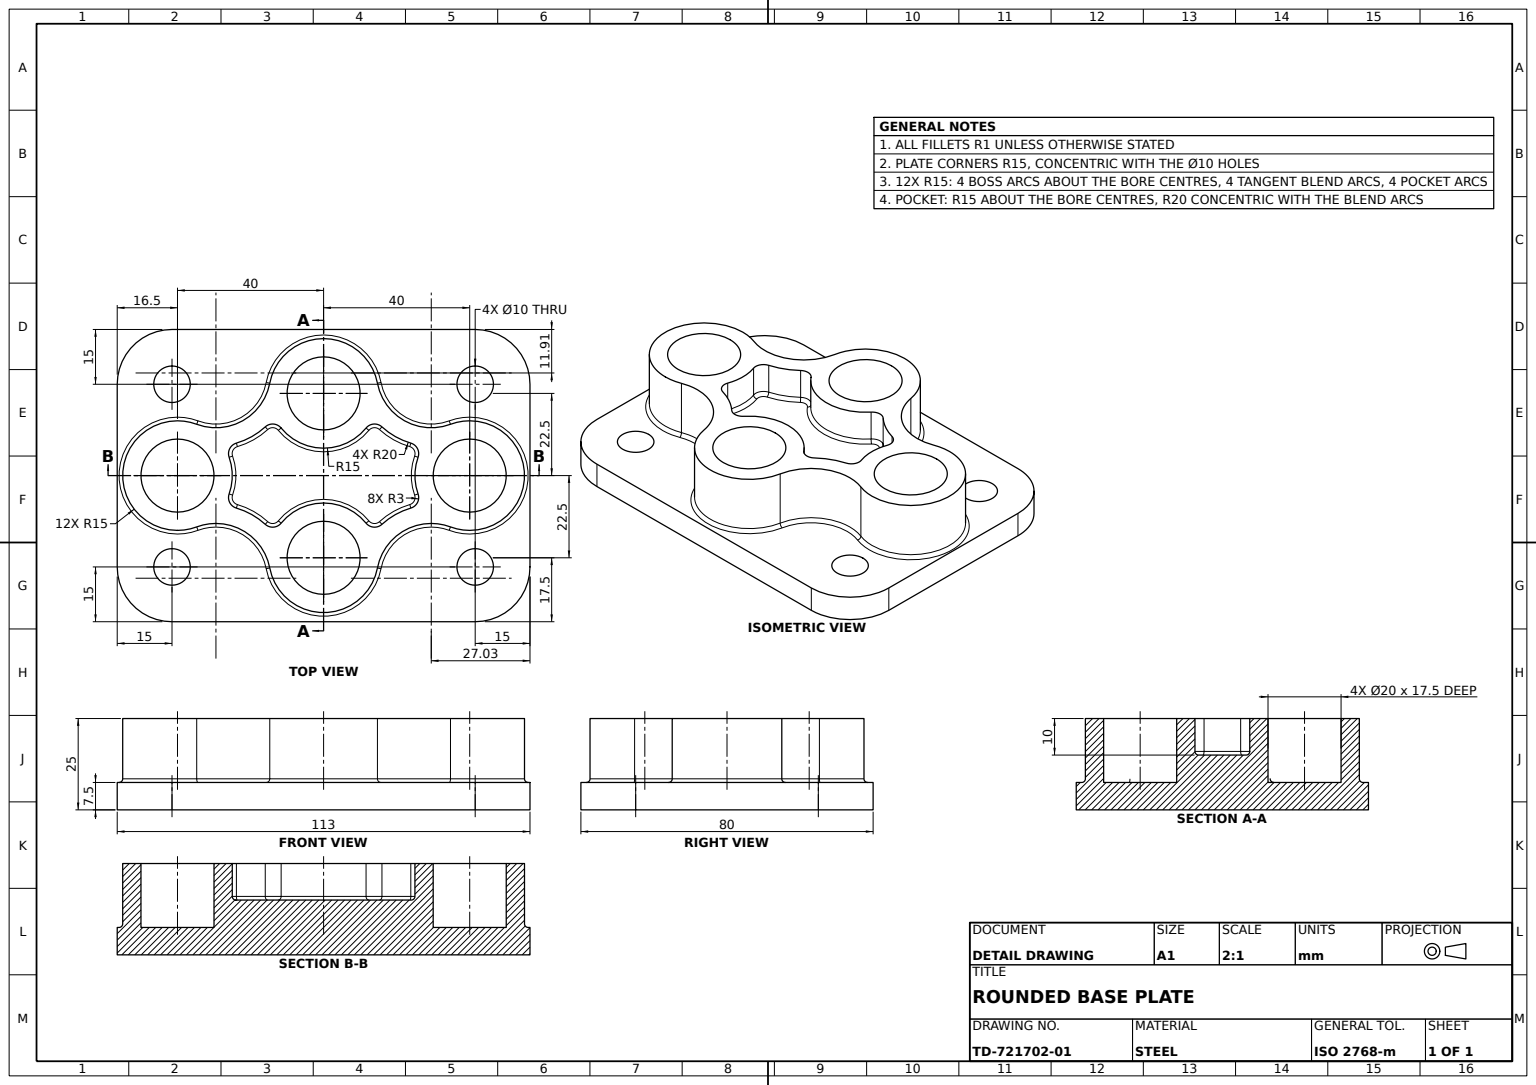
solid
v1 (-29.474069,1,13.092789)
v2 (-14.737034,1,25.296394)
e1 v1 v2 CIRCLE(AX(P(-29.474069,1,28.092789),D(0,-1,0),D(0,0,-1)),15)
v3 (-29.474069,0,14.092789)
e2 v1 v3 CIRCLE(AX(P(-29.474069,1,14.092789),D(-1,0,0),D(0,0,1)),1)
v4 (-15.719503,0,25.482821)
e3 v4 v3 CIRCLE(AX(P(-29.474069,0,28.092789),D(0,1,0),D(0,0,-1)),14)
e4 v4 v2 CIRCLE(AX(P(-15.719503,1,25.482821),D(0.186426284,0,0.982468951),D(0.982468951,0,-0.186426284)),1)
face TORUS(AX(P(-29.474069,1,28.092789),D(0,-1,0),D(0,0,-1)),14,1) rev [-e1 e2 -e3 e4]
v5 (40,1,-15)
v6 (34.737034,1,-14.046394)
e5 v5 v6 CIRCLE(AX(P(40,1,0),D(0,1,0),D(0,0,-1)),15)
v7 (34.737034,17.5,-14.046394)
e6 v7 v6 LINE
v8 (40,17.5,-15)
e7 v8 v7 CIRCLE(AX(P(40,17.5,0),D(0,1,0),D(0,0,-1)),15)
e8 v8 v5 LINE
face CYL(AX(P(40,17.5,0),D(0,-1,0),D(0,0,-1)),15) [e5 -e6 -e7 e8]
v9 (-34.737034,1,-14.046394)
v10 (-40,1,-15)
e9 v9 v10 CIRCLE(AX(P(-40,1,0),D(0,1,0),D(0,0,-1)),15)
v11 (-34.38617,0,-14.982821)
e10 v9 v11 CIRCLE(AX(P(-34.38617,1,-14.982821),D(0.936426284,0,0.350864382),D(0.350864382,0,-0.936426284)),1)
v12 (-40,0,-16)
e11 v12 v11 CIRCLE(AX(P(-40,0,0),D(0,-1,0),D(0,0,-1)),16)
e12 v12 v10 CIRCLE(AX(P(-40,1,-16),D(-1,0,0),D(0,0,1)),1)
face TORUS(AX(P(-40,1,0),D(0,-1,0),D(0,0,-1)),16,1) rev [-e9 e10 -e11 e12]
v13 (15.298823,7.5,-12.598841)
v14 (12.398933,7.5,-12.387312)
e13 v13 v14 CIRCLE(AX(P(13.9488,7.5,-11.123226),D(0,1,0),D(0,0,1)),2)
v15 (15.973835,8.5,-13.336648)
e14 v13 v15 CIRCLE(AX(P(15.298823,8.5,-12.598841),D(0.737807048,0,0.675011674),D(0.675011674,0,-0.737807048)),1)
v16 (13.9488,8.5,-14.123226)
e15 v16 v15 CIRCLE(AX(P(13.9488,8.5,-11.123226),D(0,-1,0),D(0,0,1)),3)
v17 (11.624,8.5,-13.019355)
e16 v17 v16 CIRCLE(AX(P(13.9488,8.5,-11.123226),D(0,-1,0),D(0,0,1)),3)
e17 v14 v17 CIRCLE(AX(P(12.398933,8.5,-12.387312),D(0.632042977,0,-0.774933336),D(-0.774933336,0,-0.632042977)),1)
face TORUS(AX(P(13.9488,8.5,-11.123226),D(0,1,0),D(0,0,1)),2,1) rev [-e13 e14 -e15 -e16 -e17]
v18 (14.737034,1,-25.296394)
v19 (15.719503,0,-25.482821)
e18 v18 v19 CIRCLE(AX(P(15.719503,1,-25.482821),D(0.186426284,0,0.982468951),D(0.982468951,0,-0.186426284)),1)
v20 (0,0,-38.5)
e19 v20 v19 CIRCLE(AX(P(0,0,-22.5),D(0,-1,0),D(0,0,-1)),16)
v21 (0,1,-37.5)
e20 v20 v21 CIRCLE(AX(P(0,1,-38.5),D(-1,0,0),D(0,0,1)),1)
e21 v18 v21 CIRCLE(AX(P(0,1,-22.5),D(0,1,0),D(0,0,-1)),15)
face TORUS(AX(P(0,1,-22.5),D(0,-1,0),D(0,0,-1)),16,1) rev [e18 -e19 e20 -e21]
v22 (-40,0,16)
e22 v22 v12 CIRCLE(AX(P(-40,0,0),D(0,-1,0),D(0,0,-1)),16)
v23 (-40,1,15)
e23 v22 v23 CIRCLE(AX(P(-40,1,16),D(1,0,0),D(0,0,-1)),1)
e24 v10 v23 CIRCLE(AX(P(-40,1,0),D(0,1,0),D(0,0,-1)),15)
face TORUS(AX(P(-40,1,0),D(0,-1,0),D(0,0,-1)),16,1) rev [-e22 e23 -e24 -e12]
v24 (-25.861645,17.5,-5.01068)
v25 (-25.861645,8.5,-5.01068)
e25 v24 v25 LINE
v26 (-25.861645,17.5,5.01068)
e26 v24 v26 CIRCLE(AX(P(-40,17.5,0),D(0,-1,0),D(0,0,1)),15)
v27 (-25.861645,8.5,5.01068)
e27 v26 v27 LINE
e28 v27 v25 CIRCLE(AX(P(-40,8.5,0),D(0,1,0),D(0,0,1)),15)
face CYL(AX(P(-40,17.5,0),D(0,-1,0),D(0,0,-1)),15) [-e25 e26 e27 e28]
v28 (40,17.5,15)
e29 v28 v8 CIRCLE(AX(P(40,17.5,0),D(0,1,0),D(0,0,-1)),15)
v29 (40,1,15)
e30 v28 v29 LINE
e31 v29 v5 CIRCLE(AX(P(40,1,0),D(0,1,0),D(0,0,-1)),15)
face CYL(AX(P(40,17.5,0),D(0,-1,0),D(0,0,-1)),15) [-e29 e30 e31 -e8]
v30 (56.5,0,25)
v31 (56.5,-7.5,25)
e32 v30 v31 LINE
v32 (41.5,0,40)
e33 v32 v30 CIRCLE(AX(P(41.5,0,25),D(0,1,0),D(0,0,-1)),15)
v33 (41.5,-7.5,40)
e34 v33 v32 LINE
e35 v31 v33 CIRCLE(AX(P(41.5,-7.5,25),D(0,-1,0),D(0,0,-1)),15)
face CYL(AX(P(41.5,-7.5,25),D(0,1,0),D(0,0,1)),15) [-e32 -e33 -e34 -e35]
v34 (23.593982,7.5,7.932814)
v35 (23.873986,8.5,8.892813)
e36 v34 v35 CIRCLE(AX(P(23.593982,8.5,7.932814),D(-0.9599988,0,0.280004116),D(0.280004116,0,0.9599988)),1)
v36 (25.861645,8.5,5.01068)
e37 v36 v35 CIRCLE(AX(P(23.033974,8.5,6.012816),D(0,-1,0),D(0,0,1)),3)
v37 (24.919088,7.5,5.344725)
e38 v37 v36 CIRCLE(AX(P(24.919088,8.5,5.344725),D(0.334045341,0,0.942557006),D(0.942557006,0,-0.334045341)),1)
e39 v34 v37 CIRCLE(AX(P(23.033974,7.5,6.012816),D(0,1,0),D(0,0,1)),2)
face TORUS(AX(P(23.033974,8.5,6.012816),D(0,1,0),D(0,0,1)),2,1) rev [e36 -e37 -e38 -e39]
v38 (15.719503,0,25.482821)
e40 v38 v4 CIRCLE(AX(P(0,0,22.5),D(0,-1,0),D(0,0,-1)),16)
v39 (14.737034,1,25.296394)
e41 v38 v39 CIRCLE(AX(P(15.719503,1,25.482821),D(0.186426284,0,-0.982468951),D(-0.982468951,0,-0.186426284)),1)
e42 v2 v39 CIRCLE(AX(P(0,1,22.5),D(0,1,0),D(0,0,-1)),15)
face TORUS(AX(P(0,1,22.5),D(0,-1,0),D(0,0,-1)),16,1) rev [-e40 e41 -e42 -e4]
v40 (0,17.5,-37.5)
v41 (-14.737034,17.5,-25.296394)
e43 v40 v41 CIRCLE(AX(P(0,17.5,-22.5),D(0,1,0),D(0,0,-1)),15)
e44 v40 v21 LINE
v42 (-14.737034,1,-25.296394)
e45 v21 v42 CIRCLE(AX(P(0,1,-22.5),D(0,1,0),D(0,0,-1)),15)
e46 v41 v42 LINE
face CYL(AX(P(0,17.5,-22.5),D(0,-1,0),D(0,0,-1)),15) [-e43 e44 e45 -e46]
v43 (-15.973835,8.5,-13.336648)
v44 (-13.9488,8.5,-14.123226)
e47 v43 v44 CIRCLE(AX(P(-13.9488,8.5,-11.123226),D(0,-1,0),D(0,0,1)),3)
v45 (-13.9488,17.5,-14.123226)
e48 v45 v44 LINE
v46 (-15.973835,17.5,-13.336648)
e49 v45 v46 CIRCLE(AX(P(-13.9488,17.5,-11.123226),D(0,1,0),D(0,0,1)),3)
e50 v46 v43 LINE
face CYL(AX(P(-13.9488,17.5,-11.123226),D(0,-1,0),D(0,0,-1)),3) rev [e47 -e48 e49 e50]
v47 (-23.873986,17.5,8.892813)
v48 (-23.873986,8.5,8.892813)
e51 v47 v48 LINE
v49 (-15.973835,17.5,13.336648)
e52 v47 v49 CIRCLE(AX(P(-29.474069,17.5,28.092789),D(0,-1,0),D(0,0,-1)),20)
v50 (-15.973835,8.5,13.336648)
e53 v49 v50 LINE
e54 v50 v48 CIRCLE(AX(P(-29.474069,8.5,28.092789),D(0,1,0),D(0,0,1)),20)
face CYL(AX(P(-29.474069,17.5,28.092789),D(0,-1,0),D(0,0,-1)),20) [-e51 e52 e53 e54]
v51 (-41.5,0,40)
e55 v51 v32 LINE
v52 (-41.5,-7.5,40)
e56 v51 v52 LINE
e57 v52 v33 LINE
face PLANE(AX(P(-56.5,-7.5,40),D(0,0,1),D(1,0,0))) [-e55 e56 e57 e34]
v53 (40,0,-16)
e58 v53 v5 CIRCLE(AX(P(40,1,-16),D(-1,0,0),D(0,0,1)),1)
v54 (40,0,16)
e59 v54 v29 CIRCLE(AX(P(40,1,16),D(1,0,0),D(0,0,-1)),1)
e60 v53 v54 CIRCLE(AX(P(40,0,0),D(0,-1,0),D(0,0,-1)),16)
face TORUS(AX(P(40,1,0),D(0,-1,0),D(0,0,-1)),16,1) rev [e58 -e31 -e59 -e60]
v55 (13.9488,17.5,-14.123226)
e61 v55 v16 LINE
v56 (11.624,17.5,-13.019355)
e62 v55 v56 CIRCLE(AX(P(13.9488,17.5,-11.123226),D(0,1,0),D(0,0,-1)),3)
e63 v56 v17 LINE
face CYL(AX(P(13.9488,17.5,-11.123226),D(0,-1,0),D(0,0,-1)),3) rev [e16 -e61 e62 e63]
v57 (-14.737034,17.5,25.296394)
e64 v57 v2 LINE
v58 (14.737034,17.5,25.296394)
e65 v58 v39 LINE
e66 v57 v58 CIRCLE(AX(P(0,17.5,22.5),D(0,1,0),D(0,0,1)),15)
face CYL(AX(P(0,17.5,22.5),D(0,-1,0),D(0,0,-1)),15) [e64 e42 -e65 -e66]
v59 (-29.474069,17.5,13.092789)
e67 v59 v57 CIRCLE(AX(P(-29.474069,17.5,28.092789),D(0,-1,0),D(0,0,-1)),15)
e68 v59 v1 LINE
face CYL(AX(P(-29.474069,17.5,28.092789),D(0,-1,0),D(0,0,-1)),15) rev [-e64 -e67 e68 e1]
v60 (34.737034,1,14.046394)
e69 v60 v29 CIRCLE(AX(P(40,1,0),D(0,1,0),D(0,0,-1)),15)
v61 (34.38617,0,14.982821)
e70 v61 v60 CIRCLE(AX(P(34.38617,1,14.982821),D(0.936426284,0,0.350864382),D(0.350864382,0,-0.936426284)),1)
e71 v54 v61 CIRCLE(AX(P(40,0,0),D(0,-1,0),D(0,0,-1)),16)
face TORUS(AX(P(40,1,0),D(0,-1,0),D(0,0,-1)),16,1) rev [-e69 -e70 -e71 e59]
v62 (0,0,-32.5)
v63 (0,0,-12.5)
e72 v62 v63 CIRCLE(AX(P(0,0,-22.5),D(0,1,0),D(0,0,-1)),10)
e73 v63 v62 CIRCLE(AX(P(0,0,-22.5),D(0,1,0),D(0,0,-1)),10)
face PLANE(AX(P(0,0,0),D(0,-1,0),D(0,0,-1))) rev [e72 e73]
v64 (-23.873986,8.5,-8.892813)
e74 v64 v43 CIRCLE(AX(P(-29.474069,8.5,-28.092789),D(0,1,0),D(0,0,1)),20)
v65 (-23.593982,7.5,-7.932814)
e75 v64 v65 CIRCLE(AX(P(-23.593982,8.5,-7.932814),D(-0.9599988,0,0.280004116),D(0.280004116,0,0.9599988)),1)
v66 (-15.298823,7.5,-12.598841)
e76 v66 v65 CIRCLE(AX(P(-29.474069,7.5,-28.092789),D(0,-1,0),D(0,0,1)),21)
e77 v43 v66 CIRCLE(AX(P(-15.298823,8.5,-12.598841),D(-0.737807048,0,0.675011674),D(0.675011674,0,0.737807048)),1)
face TORUS(AX(P(-29.474069,8.5,-28.092789),D(0,1,0),D(0,0,1)),21,1) rev [-e74 e75 -e76 -e77]
v67 (-41.5,0,-30)
v68 (-41.5,0,-20)
e78 v67 v68 CIRCLE(AX(P(-41.5,0,-25),D(0,1,0),D(0,0,1)),5)
v69 (-41.5,-7.5,-20)
e79 v69 v68 LINE
v70 (-41.5,-7.5,-30)
e80 v69 v70 CIRCLE(AX(P(-41.5,-7.5,-25),D(0,-1,0),D(0,0,-1)),5)
e81 v70 v67 LINE
face CYL(AX(P(-41.5,-17.5,-25),D(0,1,0),D(0,0,1)),5) rev [e78 -e79 e80 e81]
v71 (29.474069,1,13.092789)
e82 v39 v71 CIRCLE(AX(P(29.474069,1,28.092789),D(0,-1,0),D(0,0,-1)),15)
v72 (29.474069,17.5,13.092789)
e83 v72 v71 LINE
e84 v58 v72 CIRCLE(AX(P(29.474069,17.5,28.092789),D(0,-1,0),D(0,0,1)),15)
face CYL(AX(P(29.474069,17.5,28.092789),D(0,-1,0),D(0,0,-1)),15) rev [e82 -e83 -e84 e65]
v73 (40,0,10)
v74 (40,0,-10)
e85 v73 v74 CIRCLE(AX(P(40,0,0),D(0,1,0),D(0,0,-1)),10)
e86 v74 v73 CIRCLE(AX(P(40,0,0),D(0,1,0),D(0,0,-1)),10)
face PLANE(AX(P(0,0,0),D(0,-1,0),D(0,0,-1))) rev [e85 e86]
v75 (15.973835,17.5,13.336648)
v76 (15.973835,8.5,13.336648)
e87 v75 v76 LINE
v77 (23.873986,17.5,8.892813)
e88 v75 v77 CIRCLE(AX(P(29.474069,17.5,28.092789),D(0,-1,0),D(0,0,1)),20)
e89 v77 v35 LINE
e90 v35 v76 CIRCLE(AX(P(29.474069,8.5,28.092789),D(0,1,0),D(0,0,1)),20)
face CYL(AX(P(29.474069,17.5,28.092789),D(0,-1,0),D(0,0,-1)),20) [-e87 e88 e89 e90]
v78 (-24.919088,7.5,5.344725)
e91 v27 v78 CIRCLE(AX(P(-24.919088,8.5,5.344725),D(-0.334045341,0,0.942557006),D(0.942557006,0,0.334045341)),1)
v79 (-24.919088,7.5,-5.344725)
e92 v79 v78 CIRCLE(AX(P(-40,7.5,0),D(0,-1,0),D(0,0,1)),16)
e93 v25 v79 CIRCLE(AX(P(-24.919088,8.5,-5.344725),D(0.334045341,0,0.942557006),D(0.942557006,0,-0.334045341)),1)
face TORUS(AX(P(-40,8.5,0),D(0,1,0),D(0,0,1)),16,1) rev [e91 -e92 -e93 -e28]
v80 (15.298823,7.5,12.598841)
e94 v80 v76 CIRCLE(AX(P(15.298823,8.5,12.598841),D(-0.737807048,0,0.675011674),D(0.675011674,0,0.737807048)),1)
e95 v80 v34 CIRCLE(AX(P(29.474069,7.5,28.092789),D(0,-1,0),D(0,0,1)),21)
face TORUS(AX(P(29.474069,8.5,28.092789),D(0,1,0),D(0,0,1)),21,1) rev [e94 -e90 -e36 -e95]
v81 (-11.624,17.5,13.019355)
e96 v49 v81 CIRCLE(AX(P(-13.9488,17.5,11.123226),D(0,1,0),D(0,0,-1)),3)
v82 (-11.624,8.5,13.019355)
e97 v81 v82 LINE
v83 (-13.9488,8.5,14.123226)
e98 v82 v83 CIRCLE(AX(P(-13.9488,8.5,11.123226),D(0,-1,0),D(0,0,1)),3)
e99 v83 v50 CIRCLE(AX(P(-13.9488,8.5,11.123226),D(0,-1,0),D(0,0,1)),3)
face CYL(AX(P(-13.9488,17.5,11.123226),D(0,-1,0),D(0,0,-1)),3) rev [e96 e97 e98 e99 -e53]
v84 (41.5,-7.5,-20)
v85 (41.5,-7.5,-30)
e100 v84 v85 CIRCLE(AX(P(41.5,-7.5,-25),D(0,-1,0),D(0,0,-1)),5)
e101 v85 v84 CIRCLE(AX(P(41.5,-7.5,-25),D(0,-1,0),D(0,0,-1)),5)
v86 (41.5,-7.5,30)
v87 (41.5,-7.5,20)
e102 v86 v87 CIRCLE(AX(P(41.5,-7.5,25),D(0,-1,0),D(0,0,-1)),5)
e103 v87 v86 CIRCLE(AX(P(41.5,-7.5,25),D(0,-1,0),D(0,0,-1)),5)
v88 (-56.5,-7.5,-25)
v89 (-56.5,-7.5,25)
e104 v88 v89 LINE
v90 (-41.5,-7.5,-40)
e105 v88 v90 CIRCLE(AX(P(-41.5,-7.5,-25),D(0,-1,0),D(0,0,-1)),15)
v91 (41.5,-7.5,-40)
e106 v91 v90 LINE
v92 (56.5,-7.5,-25)
e107 v91 v92 CIRCLE(AX(P(41.5,-7.5,-25),D(0,-1,0),D(0,0,-1)),15)
e108 v31 v92 LINE
e109 v52 v89 CIRCLE(AX(P(-41.5,-7.5,25),D(0,-1,0),D(0,0,-1)),15)
v93 (-41.5,-7.5,30)
v94 (-41.5,-7.5,20)
e110 v93 v94 CIRCLE(AX(P(-41.5,-7.5,25),D(0,-1,0),D(0,0,-1)),5)
e111 v94 v93 CIRCLE(AX(P(-41.5,-7.5,25),D(0,-1,0),D(0,0,-1)),5)
e112 v70 v69 CIRCLE(AX(P(-41.5,-7.5,-25),D(0,-1,0),D(0,0,-1)),5)
face PLANE(AX(P(0,-7.5,0),D(0,-1,0),D(0,0,-1))) [-e100 -e101] [-e102 -e103] [-e104 e105 -e106 e107 -e108 e35 -e57 e109] [-e110 -e111] [-e112 -e80]
v95 (0,17.5,32.5)
v96 (0,17.5,12.5)
e113 v95 v96 CIRCLE(AX(P(0,17.5,22.5),D(0,1,0),D(0,0,1)),10)
v97 (0,0,12.5)
e114 v96 v97 LINE
v98 (0,0,32.5)
e115 v98 v97 CIRCLE(AX(P(0,0,22.5),D(0,1,0),D(0,0,1)),10)
e116 v95 v98 LINE
face CYL(AX(P(0,17.5,22.5),D(0,-1,0),D(0,0,-1)),10) rev [e113 e114 -e115 -e116]
v99 (-41.5,0,30)
e117 v93 v99 LINE
v100 (-41.5,0,20)
e118 v99 v100 CIRCLE(AX(P(-41.5,0,25),D(0,1,0),D(0,0,1)),5)
e119 v94 v100 LINE
face CYL(AX(P(-41.5,-17.5,25),D(0,1,0),D(0,0,1)),5) rev [e117 e118 -e119 e111]
v101 (24.919088,7.5,-5.344725)
v102 (25.861645,8.5,-5.01068)
e120 v101 v102 CIRCLE(AX(P(24.919088,8.5,-5.344725),D(-0.334045341,0,0.942557006),D(0.942557006,0,0.334045341)),1)
v103 (23.873986,8.5,-8.892813)
e121 v103 v102 CIRCLE(AX(P(23.033974,8.5,-6.012816),D(0,-1,0),D(0,0,1)),3)
v104 (23.593982,7.5,-7.932814)
e122 v104 v103 CIRCLE(AX(P(23.593982,8.5,-7.932814),D(0.9599988,0,0.280004116),D(0.280004116,0,-0.9599988)),1)
e123 v101 v104 CIRCLE(AX(P(23.033974,7.5,-6.012816),D(0,1,0),D(0,0,1)),2)
face TORUS(AX(P(23.033974,8.5,-6.012816),D(0,1,0),D(0,0,1)),2,1) rev [e120 -e121 -e122 -e123]
v105 (-15.719503,0,-25.482821)
e124 v105 v20 CIRCLE(AX(P(0,0,-22.5),D(0,-1,0),D(0,0,-1)),16)
e125 v42 v105 CIRCLE(AX(P(-15.719503,1,-25.482821),D(0.186426284,0,-0.982468951),D(-0.982468951,0,-0.186426284)),1)
face TORUS(AX(P(0,1,-22.5),D(0,-1,0),D(0,0,-1)),16,1) rev [-e124 -e125 -e45 -e20]
v106 (-23.873986,17.5,-8.892813)
e126 v46 v106 CIRCLE(AX(P(-29.474069,17.5,-28.092789),D(0,-1,0),D(0,0,1)),20)
e127 v106 v64 LINE
face CYL(AX(P(-29.474069,17.5,-28.092789),D(0,-1,0),D(0,0,-1)),20) [-e50 e126 e127 e74]
v107 (41.5,0,-20)
v108 (41.5,0,-30)
e128 v107 v108 CIRCLE(AX(P(41.5,0,-25),D(0,1,0),D(0,0,-1)),5)
e129 v85 v108 LINE
e130 v84 v107 LINE
face CYL(AX(P(41.5,-17.5,-25),D(0,1,0),D(0,0,1)),5) rev [e128 -e129 e101 e130]
v109 (-34.38617,0,14.982821)
v110 (-34.737034,1,14.046394)
e131 v109 v110 CIRCLE(AX(P(-34.38617,1,14.982821),D(0.936426284,0,-0.350864382),D(-0.350864382,0,-0.936426284)),1)
e132 v23 v110 CIRCLE(AX(P(-40,1,0),D(0,1,0),D(0,0,-1)),15)
e133 v109 v22 CIRCLE(AX(P(-40,0,0),D(0,-1,0),D(0,0,-1)),16)
face TORUS(AX(P(-40,1,0),D(0,-1,0),D(0,0,-1)),16,1) rev [e131 -e132 -e23 -e133]
v111 (0,17.5,-12.5)
e134 v111 v63 LINE
v112 (0,17.5,-32.5)
e135 v111 v112 CIRCLE(AX(P(0,17.5,-22.5),D(0,1,0),D(0,0,-1)),10)
e136 v112 v62 LINE
face CYL(AX(P(0,17.5,-22.5),D(0,-1,0),D(0,0,-1)),10) rev [-e73 -e134 e135 e136]
e137 v48 v27 CIRCLE(AX(P(-23.033974,8.5,6.012816),D(0,-1,0),D(0,0,1)),3)
e138 v26 v47 CIRCLE(AX(P(-23.033974,17.5,6.012816),D(0,1,0),D(0,0,-1)),3)
face CYL(AX(P(-23.033974,17.5,6.012816),D(0,-1,0),D(0,0,-1)),3) rev [e137 -e27 e138 e51]
v113 (12.398933,7.5,12.387312)
v114 (13.9488,7.5,13.123226)
e139 v113 v114 CIRCLE(AX(P(13.9488,7.5,11.123226),D(0,1,0),D(0,0,1)),2)
v115 (11.624,8.5,13.019355)
e140 v113 v115 CIRCLE(AX(P(12.398933,8.5,12.387312),D(-0.632042977,0,-0.774933336),D(-0.774933336,0,0.632042977)),1)
v116 (13.9488,8.5,14.123226)
e141 v116 v115 CIRCLE(AX(P(13.9488,8.5,11.123226),D(0,-1,0),D(0,0,1)),3)
e142 v114 v116 CIRCLE(AX(P(13.9488,8.5,13.123226),D(-1,0,0),D(0,0,1)),1)
face TORUS(AX(P(13.9488,8.5,11.123226),D(0,1,0),D(0,0,1)),2,1) rev [-e139 e140 -e141 -e142]
v117 (40,17.5,10)
e143 v117 v73 LINE
v118 (40,17.5,-10)
e144 v117 v118 CIRCLE(AX(P(40,17.5,0),D(0,1,0),D(0,0,-1)),10)
e145 v118 v74 LINE
face CYL(AX(P(40,17.5,0),D(0,-1,0),D(0,0,-1)),10) rev [-e143 e144 e145 -e85]
v119 (-34.737034,17.5,-14.046394)
v120 (-40,17.5,-15)
e146 v119 v120 CIRCLE(AX(P(-40,17.5,0),D(0,1,0),D(0,0,1)),15)
e147 v119 v9 LINE
e148 v120 v10 LINE
face CYL(AX(P(-40,17.5,0),D(0,-1,0),D(0,0,-1)),15) [-e146 e147 e9 -e148]
e149 v3 v109 CIRCLE(AX(P(-29.474069,0,28.092789),D(0,1,0),D(0,0,-1)),14)
e150 v110 v1 CIRCLE(AX(P(-29.474069,1,28.092789),D(0,-1,0),D(0,0,-1)),15)
face TORUS(AX(P(-29.474069,1,28.092789),D(0,-1,0),D(0,0,-1)),14,1) rev [-e131 -e149 -e2 -e150]
e151 v65 v79 CIRCLE(AX(P(-23.033974,7.5,-6.012816),D(0,1,0),D(0,0,1)),2)
e152 v25 v64 CIRCLE(AX(P(-23.033974,8.5,-6.012816),D(0,-1,0),D(0,0,1)),3)
face TORUS(AX(P(-23.033974,8.5,-6.012816),D(0,1,0),D(0,0,1)),2,1) rev [e93 -e151 -e75 -e152]
e153 v100 v99 CIRCLE(AX(P(-41.5,0,25),D(0,1,0),D(0,0,1)),5)
face CYL(AX(P(-41.5,-17.5,25),D(0,1,0),D(0,0,1)),5) rev [e110 e119 e153 -e117]
v121 (-40,17.5,15)
e154 v121 v23 LINE
v122 (-34.737034,17.5,14.046394)
e155 v122 v110 LINE
e156 v121 v122 CIRCLE(AX(P(-40,17.5,0),D(0,1,0),D(0,0,1)),15)
face CYL(AX(P(-40,17.5,0),D(0,-1,0),D(0,0,-1)),15) [e154 e132 -e155 -e156]
e157 v112 v111 CIRCLE(AX(P(0,17.5,-22.5),D(0,1,0),D(0,0,-1)),10)
face CYL(AX(P(0,17.5,-22.5),D(0,-1,0),D(0,0,-1)),10) rev [-e136 e157 e134 -e72]
e158 v15 v103 CIRCLE(AX(P(29.474069,8.5,-28.092789),D(0,1,0),D(0,0,1)),20)
e159 v104 v13 CIRCLE(AX(P(29.474069,7.5,-28.092789),D(0,-1,0),D(0,0,1)),21)
face TORUS(AX(P(29.474069,8.5,-28.092789),D(0,1,0),D(0,0,1)),21,1) rev [e122 -e158 -e14 -e159]
v123 (29.474069,0,14.092789)
e160 v71 v123 CIRCLE(AX(P(29.474069,1,14.092789),D(-1,0,0),D(0,0,1)),1)
e161 v123 v38 CIRCLE(AX(P(29.474069,0,28.092789),D(0,1,0),D(0,0,-1)),14)
face TORUS(AX(P(29.474069,1,28.092789),D(0,-1,0),D(0,0,-1)),14,1) rev [-e160 -e82 -e41 -e161]
v124 (56.5,0,-25)
e162 v92 v124 LINE
e163 v30 v124 LINE
face PLANE(AX(P(56.5,-7.5,40),D(1,0,0),D(0,0,-1))) [e108 e162 -e163 e32]
e164 v76 v116 CIRCLE(AX(P(13.9488,8.5,11.123226),D(0,-1,0),D(0,0,1)),3)
e165 v114 v80 CIRCLE(AX(P(13.9488,7.5,11.123226),D(0,1,0),D(0,0,1)),2)
face TORUS(AX(P(13.9488,8.5,11.123226),D(0,1,0),D(0,0,1)),2,1) rev [e142 -e164 -e94 -e165]
v125 (34.38617,0,-14.982821)
e166 v6 v125 CIRCLE(AX(P(34.38617,1,-14.982821),D(0.936426284,0,-0.350864382),D(-0.350864382,0,-0.936426284)),1)
e167 v19 v125 CIRCLE(AX(P(29.474069,0,-28.092789),D(0,1,0),D(0,0,-1)),14)
e168 v6 v18 CIRCLE(AX(P(29.474069,1,-28.092789),D(0,-1,0),D(0,0,-1)),15)
face TORUS(AX(P(29.474069,1,-28.092789),D(0,-1,0),D(0,0,-1)),14,1) rev [e166 -e167 -e18 -e168]
v126 (-15.298823,7.5,12.598841)
e169 v50 v126 CIRCLE(AX(P(-15.298823,8.5,12.598841),D(0.737807048,0,0.675011674),D(0.675011674,0,-0.737807048)),1)
v127 (-13.9488,7.5,13.123226)
e170 v127 v83 CIRCLE(AX(P(-13.9488,8.5,13.123226),D(-1,0,0),D(0,0,1)),1)
e171 v126 v127 CIRCLE(AX(P(-13.9488,7.5,11.123226),D(0,1,0),D(0,0,1)),2)
face TORUS(AX(P(-13.9488,8.5,11.123226),D(0,1,0),D(0,0,1)),2,1) rev [-e169 -e99 -e170 -e171]
v128 (14.737034,17.5,-25.296394)
e172 v7 v128 CIRCLE(AX(P(29.474069,17.5,-28.092789),D(0,-1,0),D(0,0,-1)),15)
e173 v128 v18 LINE
face CYL(AX(P(29.474069,17.5,-28.092789),D(0,-1,0),D(0,0,-1)),15) rev [-e172 e6 e168 -e173]
v129 (0,8.5,7.5)
e174 v129 v82 CIRCLE(AX(P(0,8.5,22.5),D(0,1,0),D(0,0,1)),15)
v130 (0,17.5,7.5)
e175 v81 v130 CIRCLE(AX(P(0,17.5,22.5),D(0,-1,0),D(0,0,1)),15)
e176 v130 v129 LINE
face CYL(AX(P(0,17.5,22.5),D(0,-1,0),D(0,0,-1)),15) [e174 -e97 e175 e176]
e177 v118 v117 CIRCLE(AX(P(40,17.5,0),D(0,1,0),D(0,0,-1)),10)
face CYL(AX(P(40,17.5,0),D(0,-1,0),D(0,0,-1)),10) rev [-e145 e177 e143 -e86]
e178 v128 v40 CIRCLE(AX(P(0,17.5,-22.5),D(0,1,0),D(0,0,-1)),15)
face CYL(AX(P(0,17.5,-22.5),D(0,-1,0),D(0,0,-1)),15) [-e44 -e178 e173 e21]
v131 (34.737034,17.5,14.046394)
e179 v131 v28 CIRCLE(AX(P(40,17.5,0),D(0,1,0),D(0,0,-1)),15)
e180 v131 v60 LINE
face CYL(AX(P(40,17.5,0),D(0,-1,0),D(0,0,-1)),15) [-e30 -e179 e180 e69]
v132 (41.5,0,-40)
e181 v132 v91 LINE
e182 v124 v132 CIRCLE(AX(P(41.5,0,-25),D(0,1,0),D(0,0,-1)),15)
face CYL(AX(P(41.5,-7.5,-25),D(0,1,0),D(0,0,1)),15) [-e162 -e107 -e181 -e182]
v133 (-40,17.5,-10)
v134 (-40,17.5,10)
e183 v133 v134 CIRCLE(AX(P(-40,17.5,0),D(0,1,0),D(0,0,1)),10)
e184 v134 v133 CIRCLE(AX(P(-40,17.5,0),D(0,1,0),D(0,0,1)),10)
v135 (15.973835,17.5,-13.336648)
e185 v135 v55 CIRCLE(AX(P(13.9488,17.5,-11.123226),D(0,1,0),D(0,0,-1)),3)
v136 (23.873986,17.5,-8.892813)
e186 v136 v135 CIRCLE(AX(P(29.474069,17.5,-28.092789),D(0,-1,0),D(0,0,-1)),20)
v137 (25.861645,17.5,-5.01068)
e187 v137 v136 CIRCLE(AX(P(23.033974,17.5,-6.012816),D(0,1,0),D(0,0,-1)),3)
v138 (25.861645,17.5,5.01068)
e188 v138 v137 CIRCLE(AX(P(40,17.5,0),D(0,-1,0),D(0,0,-1)),15)
e189 v77 v138 CIRCLE(AX(P(23.033974,17.5,6.012816),D(0,1,0),D(0,0,1)),3)
v139 (11.624,17.5,13.019355)
e190 v139 v75 CIRCLE(AX(P(13.9488,17.5,11.123226),D(0,1,0),D(0,0,1)),3)
e191 v130 v139 CIRCLE(AX(P(0,17.5,22.5),D(0,-1,0),D(0,0,1)),15)
e192 v106 v24 CIRCLE(AX(P(-23.033974,17.5,-6.012816),D(0,1,0),D(0,0,1)),3)
v140 (-11.624,17.5,-13.019355)
e193 v140 v45 CIRCLE(AX(P(-13.9488,17.5,-11.123226),D(0,1,0),D(0,0,1)),3)
e194 v56 v140 CIRCLE(AX(P(0,17.5,-22.5),D(0,-1,0),D(0,0,-1)),15)
e195 v120 v121 CIRCLE(AX(P(-40,17.5,0),D(0,1,0),D(0,0,1)),15)
e196 v122 v59 CIRCLE(AX(P(-29.474069,17.5,28.092789),D(0,-1,0),D(0,0,-1)),15)
e197 v72 v131 CIRCLE(AX(P(29.474069,17.5,28.092789),D(0,-1,0),D(0,0,1)),15)
e198 v41 v119 CIRCLE(AX(P(-29.474069,17.5,-28.092789),D(0,-1,0),D(0,0,1)),15)
e199 v96 v95 CIRCLE(AX(P(0,17.5,22.5),D(0,1,0),D(0,0,1)),10)
face PLANE(AX(P(-14.737034,17.5,25.296394),D(0,-1,0),D(0,0,-1))) rev [-e183 -e184] [-e177 -e144] [-e62 -e185 -e186 -e187 -e188 -e189 -e88 -e190 -e191 -e175 -e96 -e52 -e138 -e26 -e192 -e126 -e49 -e193 -e194] [e146 e195 e156 e196 e67 e66 e84 e197 e179 e29 e7 e172 e178 e43 e198] [-e157 -e135] [-e199 -e113]
e200 v135 v15 LINE
face CYL(AX(P(13.9488,17.5,-11.123226),D(0,-1,0),D(0,0,-1)),3) rev [-e200 e185 e61 e15]
e201 v108 v107 CIRCLE(AX(P(41.5,0,-25),D(0,1,0),D(0,0,-1)),5)
face CYL(AX(P(41.5,-17.5,-25),D(0,1,0),D(0,0,1)),5) rev [-e130 e100 e129 e201]
v141 (-56.5,0,25)
e202 v89 v141 LINE
e203 v141 v51 CIRCLE(AX(P(-41.5,0,25),D(0,1,0),D(0,0,-1)),15)
face CYL(AX(P(-41.5,-7.5,25),D(0,1,0),D(0,0,1)),15) [-e202 -e109 -e56 -e203]
v142 (-40,0,-10)
e204 v133 v142 LINE
v143 (-40,0,10)
e205 v134 v143 LINE
e206 v142 v143 CIRCLE(AX(P(-40,0,0),D(0,1,0),D(0,0,1)),10)
face CYL(AX(P(-40,17.5,0),D(0,-1,0),D(0,0,-1)),10) rev [-e204 e183 e205 -e206]
e207 v11 v105 CIRCLE(AX(P(-29.474069,0,-28.092789),D(0,1,0),D(0,0,-1)),14)
e208 v125 v53 CIRCLE(AX(P(40,0,0),D(0,-1,0),D(0,0,-1)),16)
e209 v61 v123 CIRCLE(AX(P(29.474069,0,28.092789),D(0,1,0),D(0,0,-1)),14)
v144 (41.5,0,20)
v145 (41.5,0,30)
e210 v144 v145 CIRCLE(AX(P(41.5,0,25),D(0,1,0),D(0,0,-1)),5)
e211 v145 v144 CIRCLE(AX(P(41.5,0,25),D(0,1,0),D(0,0,-1)),5)
v146 (-41.5,0,-40)
v147 (-56.5,0,-25)
e212 v146 v147 CIRCLE(AX(P(-41.5,0,-25),D(0,1,0),D(0,0,-1)),15)
e213 v147 v141 LINE
e214 v132 v146 LINE
e215 v68 v67 CIRCLE(AX(P(-41.5,0,-25),D(0,1,0),D(0,0,1)),5)
face PLANE(AX(P(0,0,0),D(0,-1,0),D(0,0,-1))) rev [e161 e40 e3 e149 e133 e22 e11 e207 e124 e19 e167 e208 e60 e71 e209] [-e210 -e211] [e212 e213 e203 e55 e33 e163 e182 e214] [-e215 -e78] [-e128 -e201] [-e118 -e153]
e216 v102 v36 CIRCLE(AX(P(40,8.5,0),D(0,1,0),D(0,0,1)),15)
e217 v37 v101 CIRCLE(AX(P(40,7.5,0),D(0,-1,0),D(0,0,1)),16)
face TORUS(AX(P(40,8.5,0),D(0,1,0),D(0,0,1)),16,1) rev [-e216 -e120 -e217 e38]
face CYL(AX(P(-23.033974,17.5,-6.012816),D(0,-1,0),D(0,0,-1)),3) rev [e152 -e127 e192 e25]
face TORUS(AX(P(40,1,0),D(0,-1,0),D(0,0,-1)),16,1) rev [-e208 -e166 -e5 -e58]
e218 v90 v146 LINE
face PLANE(AX(P(-56.5,-7.5,-40),D(0,0,-1),D(-1,0,0))) [e181 e106 e218 -e214]
e219 v97 v98 CIRCLE(AX(P(0,0,22.5),D(0,1,0),D(0,0,1)),10)
face CYL(AX(P(0,17.5,22.5),D(0,-1,0),D(0,0,-1)),10) rev [-e114 e199 e116 -e219]
e220 v87 v144 LINE
e221 v86 v145 LINE
face CYL(AX(P(41.5,-17.5,25),D(0,1,0),D(0,0,1)),5) rev [e102 e220 e210 -e221]
e222 v137 v102 LINE
e223 v136 v103 LINE
face CYL(AX(P(23.033974,17.5,-6.012816),D(0,-1,0),D(0,0,-1)),3) rev [e121 -e222 e187 e223]
e224 v71 v60 CIRCLE(AX(P(29.474069,1,28.092789),D(0,-1,0),D(0,0,-1)),15)
face CYL(AX(P(29.474069,17.5,28.092789),D(0,-1,0),D(0,0,-1)),15) rev [e83 e224 -e180 -e197]
v148 (0,7.5,-6.5)
e225 v14 v148 CIRCLE(AX(P(0,7.5,-22.5),D(0,-1,0),D(0,0,1)),16)
v149 (-12.398933,7.5,-12.387312)
e226 v148 v149 CIRCLE(AX(P(0,7.5,-22.5),D(0,-1,0),D(0,0,1)),16)
e227 v149 v66 CIRCLE(AX(P(-13.9488,7.5,-11.123226),D(0,1,0),D(0,0,1)),2)
v150 (-23.593982,7.5,7.932814)
e228 v78 v150 CIRCLE(AX(P(-23.033974,7.5,6.012816),D(0,1,0),D(0,0,1)),2)
e229 v150 v126 CIRCLE(AX(P(-29.474069,7.5,28.092789),D(0,-1,0),D(0,0,1)),21)
v151 (-12.398933,7.5,12.387312)
e230 v127 v151 CIRCLE(AX(P(-13.9488,7.5,11.123226),D(0,1,0),D(0,0,1)),2)
e231 v151 v113 CIRCLE(AX(P(0,7.5,22.5),D(0,-1,0),D(0,0,1)),16)
face PLANE(AX(P(-26.254021,7.5,17.052802),D(0,1,0),D(0,0,1))) [e217 e123 e159 e13 e225 e226 e227 e76 e151 e92 e228 e229 e171 e230 e231 e139 e165 e95 e39]
v152 (-11.624,8.5,-13.019355)
v153 (0,8.5,-7.5)
e232 v152 v153 CIRCLE(AX(P(0,8.5,-22.5),D(0,1,0),D(0,0,1)),15)
e233 v152 v149 CIRCLE(AX(P(-12.398933,8.5,-12.387312),D(-0.632042977,0,-0.774933336),D(-0.774933336,0,0.632042977)),1)
e234 v153 v148 CIRCLE(AX(P(0,8.5,-6.5),D(-1,0,0),D(0,0,1)),1)
face TORUS(AX(P(0,8.5,-22.5),D(0,1,0),D(0,0,1)),16,1) rev [-e232 e233 -e226 -e234]
e235 v147 v88 LINE
face PLANE(AX(P(-56.5,-7.5,40),D(-1,0,0),D(0,0,1))) [e104 e202 -e213 e235]
e236 v138 v36 LINE
face CYL(AX(P(40,17.5,0),D(0,-1,0),D(0,0,-1)),15) [-e236 e188 e222 e216]
face CYL(AX(P(29.474069,17.5,-28.092789),D(0,-1,0),D(0,0,-1)),20) [e186 e200 e158 -e223]
e237 v143 v142 CIRCLE(AX(P(-40,0,0),D(0,1,0),D(0,0,1)),10)
face PLANE(AX(P(0,0,0),D(0,-1,0),D(0,0,-1))) rev [e206 e237]
e238 v42 v9 CIRCLE(AX(P(-29.474069,1,-28.092789),D(0,-1,0),D(0,0,-1)),15)
face CYL(AX(P(-29.474069,17.5,-28.092789),D(0,-1,0),D(0,0,-1)),15) rev [e46 e238 -e147 -e198]
e239 v139 v115 LINE
face CYL(AX(P(13.9488,17.5,11.123226),D(0,-1,0),D(0,0,-1)),3) rev [e190 e87 e164 e141 -e239]
face CYL(AX(P(23.033974,17.5,6.012816),D(0,-1,0),D(0,0,-1)),3) rev [e37 -e89 e189 e236]
e240 v153 v17 CIRCLE(AX(P(0,8.5,-22.5),D(0,1,0),D(0,0,1)),15)
face TORUS(AX(P(0,8.5,-22.5),D(0,1,0),D(0,0,1)),16,1) rev [-e225 e17 -e240 e234]
face CYL(AX(P(-40,17.5,0),D(0,-1,0),D(0,0,-1)),15) [-e154 -e195 e148 e24]
face CYL(AX(P(-40,17.5,0),D(0,-1,0),D(0,0,-1)),10) rev [e204 -e237 -e205 e184]
face TORUS(AX(P(-29.474069,1,-28.092789),D(0,-1,0),D(0,0,-1)),14,1) rev [-e238 e125 -e207 -e10]
face PLANE(AX(P(0,0,0),D(0,-1,0),D(0,0,-1))) rev [e115 e219]
face CYL(AX(P(-41.5,-7.5,-25),D(0,1,0),D(0,0,1)),15) [-e218 -e105 -e235 -e212]
e241 v82 v151 CIRCLE(AX(P(-12.398933,8.5,12.387312),D(0.632042977,0,-0.774933336),D(-0.774933336,0,-0.632042977)),1)
e242 v115 v129 CIRCLE(AX(P(0,8.5,22.5),D(0,1,0),D(0,0,1)),15)
face TORUS(AX(P(0,8.5,22.5),D(0,1,0),D(0,0,1)),16,1) rev [-e231 -e241 -e174 -e242 -e140]
e243 v44 v152 CIRCLE(AX(P(-13.9488,8.5,-11.123226),D(0,-1,0),D(0,0,1)),3)
e244 v140 v152 LINE
face CYL(AX(P(-13.9488,17.5,-11.123226),D(0,-1,0),D(0,0,-1)),3) rev [e193 e48 e243 -e244]
face CYL(AX(P(-41.5,-17.5,-25),D(0,1,0),D(0,0,1)),5) rev [e215 -e81 e112 e79]
face TORUS(AX(P(-13.9488,8.5,-11.123226),D(0,1,0),D(0,0,1)),2,1) rev [e77 -e227 -e233 -e243 -e47]
face CYL(AX(P(-29.474069,17.5,28.092789),D(0,-1,0),D(0,0,-1)),15) rev [e155 e150 -e68 -e196]
face TORUS(AX(P(29.474069,1,28.092789),D(0,-1,0),D(0,0,-1)),14,1) rev [-e209 e70 -e224 e160]
face CYL(AX(P(0,17.5,22.5),D(0,-1,0),D(0,0,-1)),15) [e239 e242 -e176 e191]
face TORUS(AX(P(-13.9488,8.5,11.123226),D(0,1,0),D(0,0,1)),2,1) rev [e241 -e230 e170 -e98]
e245 v48 v150 CIRCLE(AX(P(-23.593982,8.5,7.932814),D(0.9599988,0,0.280004116),D(0.280004116,0,-0.9599988)),1)
face TORUS(AX(P(-29.474069,8.5,28.092789),D(0,1,0),D(0,0,1)),21,1) rev [-e245 -e54 e169 -e229]
face CYL(AX(P(41.5,-17.5,25),D(0,1,0),D(0,0,1)),5) rev [e211 -e220 e103 e221]
face TORUS(AX(P(-23.033974,8.5,6.012816),D(0,1,0),D(0,0,1)),2,1) rev [-e137 e245 -e228 -e91]
face CYL(AX(P(0,17.5,-22.5),D(0,-1,0),D(0,0,-1)),15) [e240 -e63 e194 e244 e232]
